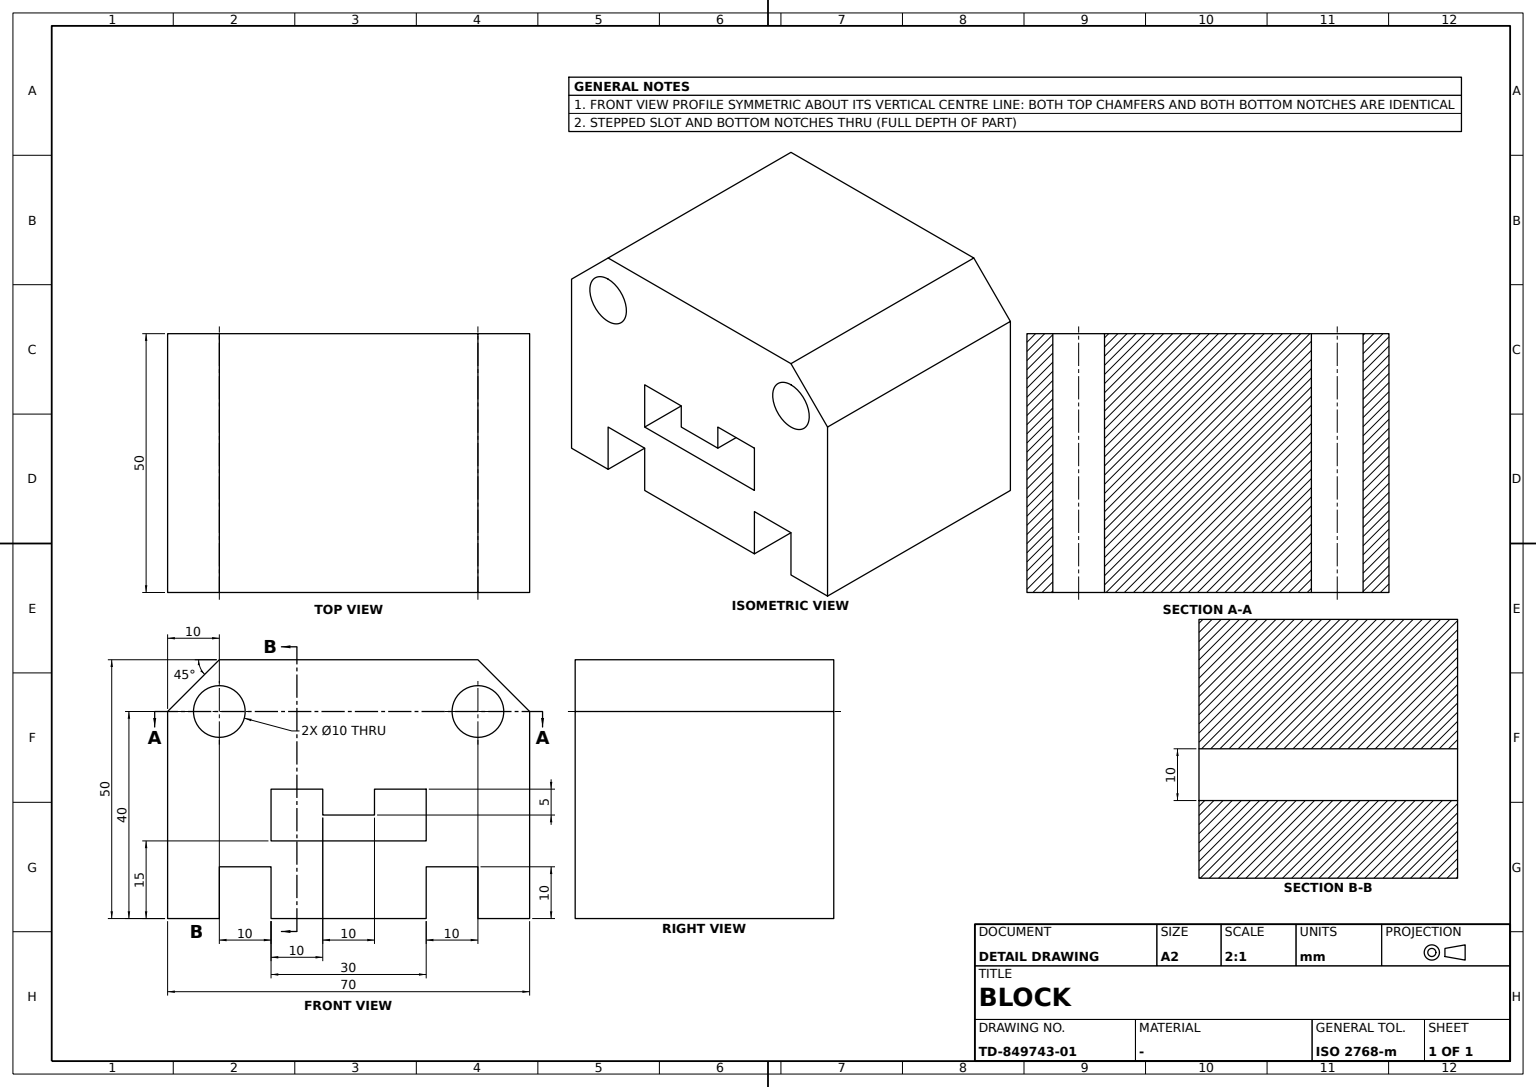
ISO-10303-21;
HEADER;
FILE_DESCRIPTION((''),'2;1');
FILE_NAME('','',(''),(''),'','','');
FILE_SCHEMA(('AUTOMOTIVE_DESIGN'));
ENDSEC;
DATA;
#1=APPLICATION_CONTEXT('');
#2=PRODUCT_CONTEXT('',#1,'mechanical');
#3=PRODUCT('','','',(#2));
#4=PRODUCT_DEFINITION_FORMATION('','',#3);
#5=PRODUCT_DEFINITION_CONTEXT('',#1,'design');
#6=PRODUCT_DEFINITION('','',#4,#5);
#7=PRODUCT_DEFINITION_SHAPE('','',#6);
#8=(LENGTH_UNIT()NAMED_UNIT(*)SI_UNIT(.MILLI.,.METRE.));
#9=(NAMED_UNIT(*)PLANE_ANGLE_UNIT()SI_UNIT($,.RADIAN.));
#10=(NAMED_UNIT(*)SI_UNIT($,.STERADIAN.)SOLID_ANGLE_UNIT());
#11=UNCERTAINTY_MEASURE_WITH_UNIT(LENGTH_MEASURE(0.005),#8,'distance_accuracy_value','');
#12=(GEOMETRIC_REPRESENTATION_CONTEXT(3)GLOBAL_UNCERTAINTY_ASSIGNED_CONTEXT((#11))GLOBAL_UNIT_ASSIGNED_CONTEXT((#8,#9,#10))REPRESENTATION_CONTEXT('',''));
#13=CARTESIAN_POINT('',(-35.,25.,0.));
#14=VERTEX_POINT('',#13);
#15=CARTESIAN_POINT('',(-35.,-25.,0.));
#16=VERTEX_POINT('',#15);
#17=CARTESIAN_POINT('',(-35.,0.,0.));
#18=DIRECTION('',(0.,-1.,0.));
#19=VECTOR('',#18,1000.);
#20=LINE('',#17,#19);
#21=EDGE_CURVE('',#14,#16,#20,.T.);
#22=ORIENTED_EDGE('',*,*,#21,.F.);
#23=CARTESIAN_POINT('',(-25.,25.,0.));
#24=VERTEX_POINT('',#23);
#25=CARTESIAN_POINT('',(0.,25.,0.));
#26=DIRECTION('',(1.,0.,0.));
#27=VECTOR('',#26,1000.);
#28=LINE('',#25,#27);
#29=EDGE_CURVE('',#14,#24,#28,.T.);
#30=ORIENTED_EDGE('',*,*,#29,.T.);
#31=CARTESIAN_POINT('',(-25.,-25.,0.));
#32=VERTEX_POINT('',#31);
#33=CARTESIAN_POINT('',(-25.,0.,0.));
#34=LINE('',#33,#19);
#35=EDGE_CURVE('',#24,#32,#34,.T.);
#36=ORIENTED_EDGE('',*,*,#35,.T.);
#37=CARTESIAN_POINT('',(0.,-25.,0.));
#38=DIRECTION('',(-1.,0.,0.));
#39=VECTOR('',#38,1000.);
#40=LINE('',#37,#39);
#41=EDGE_CURVE('',#32,#16,#40,.T.);
#42=ORIENTED_EDGE('',*,*,#41,.T.);
#43=EDGE_LOOP('',(#22,#30,#36,#42));
#44=FACE_BOUND('',#43,.T.);
#45=CARTESIAN_POINT('',(0.,0.,0.));
#46=DIRECTION('',(0.,0.,1.));
#47=AXIS2_PLACEMENT_3D('',#45,#46,#26);
#48=PLANE('',#47);
#49=ADVANCED_FACE('',(#44),#48,.F.);
#50=CARTESIAN_POINT('',(-15.,25.,15.));
#51=VERTEX_POINT('',#50);
#52=CARTESIAN_POINT('',(-15.,25.,25.));
#53=VERTEX_POINT('',#52);
#54=CARTESIAN_POINT('',(-15.,25.,0.));
#55=VECTOR('',#46,1000.);
#56=LINE('',#54,#55);
#57=EDGE_CURVE('',#51,#53,#56,.T.);
#58=ORIENTED_EDGE('',*,*,#57,.T.);
#59=CARTESIAN_POINT('',(-15.,-25.,25.));
#60=VERTEX_POINT('',#59);
#61=LINE('',#52,#19);
#62=EDGE_CURVE('',#53,#60,#61,.T.);
#63=ORIENTED_EDGE('',*,*,#62,.T.);
#64=CARTESIAN_POINT('',(-15.,-25.,15.));
#65=VERTEX_POINT('',#64);
#66=CARTESIAN_POINT('',(-15.,-25.,0.));
#67=LINE('',#66,#55);
#68=EDGE_CURVE('',#65,#60,#67,.T.);
#69=ORIENTED_EDGE('',*,*,#68,.F.);
#70=LINE('',#50,#19);
#71=EDGE_CURVE('',#51,#65,#70,.T.);
#72=ORIENTED_EDGE('',*,*,#71,.F.);
#73=EDGE_LOOP('',(#58,#63,#69,#72));
#74=FACE_BOUND('',#73,.T.);
#75=AXIS2_PLACEMENT_3D('',#54,#26,#46);
#76=PLANE('',#75);
#77=ADVANCED_FACE('',(#74),#76,.T.);
#78=CARTESIAN_POINT('',(-5.,-25.,25.));
#79=VERTEX_POINT('',#78);
#80=CARTESIAN_POINT('',(-5.,-25.,20.));
#81=VERTEX_POINT('',#80);
#82=DIRECTION('',(0.,0.,-1.));
#83=VECTOR('',#82,1000.);
#84=LINE('',#78,#83);
#85=EDGE_CURVE('',#79,#81,#84,.T.);
#86=ORIENTED_EDGE('',*,*,#85,.F.);
#87=CARTESIAN_POINT('',(-5.,25.,25.));
#88=VERTEX_POINT('',#87);
#89=LINE('',#87,#19);
#90=EDGE_CURVE('',#88,#79,#89,.T.);
#91=ORIENTED_EDGE('',*,*,#90,.F.);
#92=CARTESIAN_POINT('',(-5.,25.,20.));
#93=VERTEX_POINT('',#92);
#94=CARTESIAN_POINT('',(-5.,25.,0.));
#95=LINE('',#94,#83);
#96=EDGE_CURVE('',#88,#93,#95,.T.);
#97=ORIENTED_EDGE('',*,*,#96,.T.);
#98=LINE('',#92,#19);
#99=EDGE_CURVE('',#93,#81,#98,.T.);
#100=ORIENTED_EDGE('',*,*,#99,.T.);
#101=EDGE_LOOP('',(#86,#91,#97,#100));
#102=FACE_BOUND('',#101,.T.);
#103=AXIS2_PLACEMENT_3D('',#87,#38,#82);
#104=PLANE('',#103);
#105=ADVANCED_FACE('',(#102),#104,.T.);
#106=VERTEX_POINT('',#54);
#107=VERTEX_POINT('',#66);
#108=LINE('',#54,#19);
#109=EDGE_CURVE('',#106,#107,#108,.T.);
#110=ORIENTED_EDGE('',*,*,#109,.T.);
#111=CARTESIAN_POINT('',(-15.,-25.,10.));
#112=VERTEX_POINT('',#111);
#113=EDGE_CURVE('',#107,#112,#67,.T.);
#114=ORIENTED_EDGE('',*,*,#113,.T.);
#115=CARTESIAN_POINT('',(-15.,25.,10.));
#116=VERTEX_POINT('',#115);
#117=LINE('',#115,#19);
#118=EDGE_CURVE('',#116,#112,#117,.T.);
#119=ORIENTED_EDGE('',*,*,#118,.F.);
#120=EDGE_CURVE('',#106,#116,#56,.T.);
#121=ORIENTED_EDGE('',*,*,#120,.F.);
#122=EDGE_LOOP('',(#110,#114,#119,#121));
#123=FACE_BOUND('',#122,.T.);
#124=ADVANCED_FACE('',(#123),#76,.F.);
#125=CARTESIAN_POINT('',(25.,25.,50.));
#126=VERTEX_POINT('',#125);
#127=CARTESIAN_POINT('',(35.,25.,40.));
#128=VERTEX_POINT('',#127);
#129=CARTESIAN_POINT('',(20.,25.,55.));
#130=DIRECTION('',(0.707106781,0.,-0.707106781));
#131=VECTOR('',#130,1000.);
#132=LINE('',#129,#131);
#133=EDGE_CURVE('',#126,#128,#132,.T.);
#134=ORIENTED_EDGE('',*,*,#133,.F.);
#135=CARTESIAN_POINT('',(25.,-25.,50.));
#136=VERTEX_POINT('',#135);
#137=CARTESIAN_POINT('',(25.,0.,50.));
#138=LINE('',#137,#19);
#139=EDGE_CURVE('',#126,#136,#138,.T.);
#140=ORIENTED_EDGE('',*,*,#139,.T.);
#141=CARTESIAN_POINT('',(35.,-25.,40.));
#142=VERTEX_POINT('',#141);
#143=CARTESIAN_POINT('',(55.,-25.,20.));
#144=DIRECTION('',(-0.707106781,0.,0.707106781));
#145=VECTOR('',#144,1000.);
#146=LINE('',#143,#145);
#147=EDGE_CURVE('',#142,#136,#146,.T.);
#148=ORIENTED_EDGE('',*,*,#147,.F.);
#149=CARTESIAN_POINT('',(35.,35.,40.));
#150=LINE('',#149,#19);
#151=EDGE_CURVE('',#128,#142,#150,.T.);
#152=ORIENTED_EDGE('',*,*,#151,.F.);
#153=EDGE_LOOP('',(#134,#140,#148,#152));
#154=FACE_BOUND('',#153,.T.);
#155=DIRECTION('',(-0.707106781,0.,-0.707106781));
#156=AXIS2_PLACEMENT_3D('',#149,#155,#18);
#157=PLANE('',#156);
#158=ADVANCED_FACE('',(#154),#157,.F.);
#159=CARTESIAN_POINT('',(25.,25.,0.));
#160=VERTEX_POINT('',#159);
#161=CARTESIAN_POINT('',(35.,25.,0.));
#162=VERTEX_POINT('',#161);
#163=EDGE_CURVE('',#160,#162,#28,.T.);
#164=ORIENTED_EDGE('',*,*,#163,.T.);
#165=CARTESIAN_POINT('',(35.,-25.,0.));
#166=VERTEX_POINT('',#165);
#167=CARTESIAN_POINT('',(35.,0.,0.));
#168=DIRECTION('',(0.,1.,0.));
#169=VECTOR('',#168,1000.);
#170=LINE('',#167,#169);
#171=EDGE_CURVE('',#166,#162,#170,.T.);
#172=ORIENTED_EDGE('',*,*,#171,.F.);
#173=CARTESIAN_POINT('',(25.,-25.,0.));
#174=VERTEX_POINT('',#173);
#175=EDGE_CURVE('',#166,#174,#40,.T.);
#176=ORIENTED_EDGE('',*,*,#175,.T.);
#177=LINE('',#159,#19);
#178=EDGE_CURVE('',#160,#174,#177,.T.);
#179=ORIENTED_EDGE('',*,*,#178,.F.);
#180=EDGE_LOOP('',(#164,#172,#176,#179));
#181=FACE_BOUND('',#180,.T.);
#182=ADVANCED_FACE('',(#181),#48,.F.);
#183=CARTESIAN_POINT('',(-25.,25.,10.));
#184=VERTEX_POINT('',#183);
#185=CARTESIAN_POINT('',(-25.,-25.,10.));
#186=VERTEX_POINT('',#185);
#187=LINE('',#183,#19);
#188=EDGE_CURVE('',#184,#186,#187,.T.);
#189=ORIENTED_EDGE('',*,*,#188,.F.);
#190=CARTESIAN_POINT('',(-35.,25.,10.));
#191=LINE('',#190,#39);
#192=EDGE_CURVE('',#116,#184,#191,.T.);
#193=ORIENTED_EDGE('',*,*,#192,.F.);
#194=ORIENTED_EDGE('',*,*,#118,.T.);
#195=CARTESIAN_POINT('',(25.,-25.,10.));
#196=LINE('',#195,#39);
#197=EDGE_CURVE('',#112,#186,#196,.T.);
#198=ORIENTED_EDGE('',*,*,#197,.T.);
#199=EDGE_LOOP('',(#189,#193,#194,#198));
#200=FACE_BOUND('',#199,.T.);
#201=CARTESIAN_POINT('',(25.,25.,10.));
#202=AXIS2_PLACEMENT_3D('',#201,#46,#38);
#203=PLANE('',#202);
#204=ADVANCED_FACE('',(#200),#203,.F.);
#205=CARTESIAN_POINT('',(-35.,25.,40.));
#206=VERTEX_POINT('',#205);
#207=CARTESIAN_POINT('',(-25.,25.,50.));
#208=VERTEX_POINT('',#207);
#209=CARTESIAN_POINT('',(-55.,25.,20.));
#210=DIRECTION('',(0.707106781,0.,0.707106781));
#211=VECTOR('',#210,1000.);
#212=LINE('',#209,#211);
#213=EDGE_CURVE('',#206,#208,#212,.T.);
#214=ORIENTED_EDGE('',*,*,#213,.F.);
#215=CARTESIAN_POINT('',(-35.,-25.,40.));
#216=VERTEX_POINT('',#215);
#217=CARTESIAN_POINT('',(-35.,-35.,40.));
#218=LINE('',#217,#169);
#219=EDGE_CURVE('',#216,#206,#218,.T.);
#220=ORIENTED_EDGE('',*,*,#219,.F.);
#221=CARTESIAN_POINT('',(-25.,-25.,50.));
#222=VERTEX_POINT('',#221);
#223=CARTESIAN_POINT('',(-20.,-25.,55.));
#224=VECTOR('',#155,1000.);
#225=LINE('',#223,#224);
#226=EDGE_CURVE('',#222,#216,#225,.T.);
#227=ORIENTED_EDGE('',*,*,#226,.F.);
#228=CARTESIAN_POINT('',(-25.,0.,50.));
#229=LINE('',#228,#169);
#230=EDGE_CURVE('',#222,#208,#229,.T.);
#231=ORIENTED_EDGE('',*,*,#230,.T.);
#232=EDGE_LOOP('',(#214,#220,#227,#231));
#233=FACE_BOUND('',#232,.T.);
#234=AXIS2_PLACEMENT_3D('',#217,#130,#168);
#235=PLANE('',#234);
#236=ADVANCED_FACE('',(#233),#235,.F.);
#237=CARTESIAN_POINT('',(5.,25.,25.));
#238=VERTEX_POINT('',#237);
#239=CARTESIAN_POINT('',(5.,-25.,25.));
#240=VERTEX_POINT('',#239);
#241=LINE('',#237,#19);
#242=EDGE_CURVE('',#238,#240,#241,.T.);
#243=ORIENTED_EDGE('',*,*,#242,.F.);
#244=CARTESIAN_POINT('',(15.,25.,25.));
#245=VERTEX_POINT('',#244);
#246=CARTESIAN_POINT('',(-35.,25.,25.));
#247=LINE('',#246,#27);
#248=EDGE_CURVE('',#238,#245,#247,.T.);
#249=ORIENTED_EDGE('',*,*,#248,.T.);
#250=CARTESIAN_POINT('',(15.,-25.,25.));
#251=VERTEX_POINT('',#250);
#252=LINE('',#244,#19);
#253=EDGE_CURVE('',#245,#251,#252,.T.);
#254=ORIENTED_EDGE('',*,*,#253,.T.);
#255=LINE('',#59,#27);
#256=EDGE_CURVE('',#240,#251,#255,.T.);
#257=ORIENTED_EDGE('',*,*,#256,.F.);
#258=EDGE_LOOP('',(#243,#249,#254,#257));
#259=FACE_BOUND('',#258,.T.);
#260=AXIS2_PLACEMENT_3D('',#52,#82,#26);
#261=PLANE('',#260);
#262=ADVANCED_FACE('',(#259),#261,.T.);
#263=EDGE_CURVE('',#53,#88,#247,.T.);
#264=ORIENTED_EDGE('',*,*,#263,.F.);
#265=ORIENTED_EDGE('',*,*,#57,.F.);
#266=CARTESIAN_POINT('',(15.,25.,15.));
#267=VERTEX_POINT('',#266);
#268=CARTESIAN_POINT('',(-35.,25.,15.));
#269=LINE('',#268,#39);
#270=EDGE_CURVE('',#267,#51,#269,.T.);
#271=ORIENTED_EDGE('',*,*,#270,.F.);
#272=CARTESIAN_POINT('',(15.,25.,0.));
#273=LINE('',#272,#83);
#274=EDGE_CURVE('',#245,#267,#273,.T.);
#275=ORIENTED_EDGE('',*,*,#274,.F.);
#276=ORIENTED_EDGE('',*,*,#248,.F.);
#277=CARTESIAN_POINT('',(5.,25.,20.));
#278=VERTEX_POINT('',#277);
#279=CARTESIAN_POINT('',(5.,25.,0.));
#280=LINE('',#279,#55);
#281=EDGE_CURVE('',#278,#238,#280,.T.);
#282=ORIENTED_EDGE('',*,*,#281,.F.);
#283=CARTESIAN_POINT('',(-35.,25.,20.));
#284=LINE('',#283,#27);
#285=EDGE_CURVE('',#93,#278,#284,.T.);
#286=ORIENTED_EDGE('',*,*,#285,.F.);
#287=ORIENTED_EDGE('',*,*,#96,.F.);
#288=EDGE_LOOP('',(#264,#265,#271,#275,#276,#282,#286,#287));
#289=FACE_BOUND('',#288,.T.);
#290=CARTESIAN_POINT('',(-25.,25.,35.));
#291=VERTEX_POINT('',#290);
#292=CARTESIAN_POINT('',(-25.,25.,40.));
#293=AXIS2_PLACEMENT_3D('',#292,#18,#82);
#294=CIRCLE('',#293,5.);
#295=EDGE_CURVE('',#291,#291,#294,.F.);
#296=ORIENTED_EDGE('',*,*,#295,.F.);
#297=EDGE_LOOP('',(#296));
#298=FACE_BOUND('',#297,.T.);
#299=VERTEX_POINT('',#272);
#300=EDGE_CURVE('',#106,#299,#28,.T.);
#301=ORIENTED_EDGE('',*,*,#300,.F.);
#302=ORIENTED_EDGE('',*,*,#120,.T.);
#303=ORIENTED_EDGE('',*,*,#192,.T.);
#304=LINE('',#23,#83);
#305=EDGE_CURVE('',#184,#24,#304,.T.);
#306=ORIENTED_EDGE('',*,*,#305,.T.);
#307=ORIENTED_EDGE('',*,*,#29,.F.);
#308=LINE('',#13,#55);
#309=EDGE_CURVE('',#14,#206,#308,.T.);
#310=ORIENTED_EDGE('',*,*,#309,.T.);
#311=ORIENTED_EDGE('',*,*,#213,.T.);
#312=CARTESIAN_POINT('',(0.,25.,50.));
#313=LINE('',#312,#27);
#314=EDGE_CURVE('',#208,#126,#313,.T.);
#315=ORIENTED_EDGE('',*,*,#314,.T.);
#316=ORIENTED_EDGE('',*,*,#133,.T.);
#317=LINE('',#161,#55);
#318=EDGE_CURVE('',#162,#128,#317,.T.);
#319=ORIENTED_EDGE('',*,*,#318,.F.);
#320=ORIENTED_EDGE('',*,*,#163,.F.);
#321=VERTEX_POINT('',#201);
#322=LINE('',#159,#55);
#323=EDGE_CURVE('',#160,#321,#322,.T.);
#324=ORIENTED_EDGE('',*,*,#323,.T.);
#325=CARTESIAN_POINT('',(15.,25.,10.));
#326=VERTEX_POINT('',#325);
#327=EDGE_CURVE('',#321,#326,#191,.T.);
#328=ORIENTED_EDGE('',*,*,#327,.T.);
#329=EDGE_CURVE('',#326,#299,#273,.T.);
#330=ORIENTED_EDGE('',*,*,#329,.T.);
#331=EDGE_LOOP('',(#301,#302,#303,#306,#307,#310,#311,#315,#316,#319,#320,#324,#328,#330));
#332=FACE_BOUND('',#331,.T.);
#333=CARTESIAN_POINT('',(25.,25.,35.));
#334=VERTEX_POINT('',#333);
#335=CARTESIAN_POINT('',(25.,25.,40.));
#336=AXIS2_PLACEMENT_3D('',#335,#18,#82);
#337=CIRCLE('',#336,5.);
#338=EDGE_CURVE('',#334,#334,#337,.F.);
#339=ORIENTED_EDGE('',*,*,#338,.F.);
#340=EDGE_LOOP('',(#339));
#341=FACE_BOUND('',#340,.T.);
#342=AXIS2_PLACEMENT_3D('',#13,#18,#26);
#343=PLANE('',#342);
#344=ADVANCED_FACE('',(#289,#298,#332,#341),#343,.F.);
#345=VERTEX_POINT('',#195);
#346=CARTESIAN_POINT('',(15.,-25.,10.));
#347=VERTEX_POINT('',#346);
#348=EDGE_CURVE('',#345,#347,#196,.T.);
#349=ORIENTED_EDGE('',*,*,#348,.T.);
#350=LINE('',#325,#19);
#351=EDGE_CURVE('',#326,#347,#350,.T.);
#352=ORIENTED_EDGE('',*,*,#351,.F.);
#353=ORIENTED_EDGE('',*,*,#327,.F.);
#354=LINE('',#201,#19);
#355=EDGE_CURVE('',#321,#345,#354,.T.);
#356=ORIENTED_EDGE('',*,*,#355,.T.);
#357=EDGE_LOOP('',(#349,#352,#353,#356));
#358=FACE_BOUND('',#357,.T.);
#359=ADVANCED_FACE('',(#358),#203,.F.);
#360=CARTESIAN_POINT('',(-25.,-25.,45.));
#361=VERTEX_POINT('',#360);
#362=CARTESIAN_POINT('',(-25.,-25.,40.));
#363=AXIS2_PLACEMENT_3D('',#362,#168,#46);
#364=CIRCLE('',#363,5.);
#365=EDGE_CURVE('',#361,#361,#364,.T.);
#366=ORIENTED_EDGE('',*,*,#365,.F.);
#367=EDGE_LOOP('',(#366));
#368=FACE_BOUND('',#367,.T.);
#369=ORIENTED_EDGE('',*,*,#295,.T.);
#370=EDGE_LOOP('',(#369));
#371=FACE_BOUND('',#370,.T.);
#372=CARTESIAN_POINT('',(-25.,-0.66,40.));
#373=AXIS2_PLACEMENT_3D('',#372,#168,#38);
#374=CYLINDRICAL_SURFACE('',#373,5.);
#375=ADVANCED_FACE('',(#368,#371),#374,.F.);
#376=ORIENTED_EDGE('',*,*,#263,.T.);
#377=ORIENTED_EDGE('',*,*,#90,.T.);
#378=EDGE_CURVE('',#60,#79,#255,.T.);
#379=ORIENTED_EDGE('',*,*,#378,.F.);
#380=ORIENTED_EDGE('',*,*,#62,.F.);
#381=EDGE_LOOP('',(#376,#377,#379,#380));
#382=FACE_BOUND('',#381,.T.);
#383=ADVANCED_FACE('',(#382),#261,.T.);
#384=CARTESIAN_POINT('',(15.,-25.,0.));
#385=VERTEX_POINT('',#384);
#386=LINE('',#384,#55);
#387=EDGE_CURVE('',#385,#347,#386,.T.);
#388=ORIENTED_EDGE('',*,*,#387,.F.);
#389=CARTESIAN_POINT('',(15.,0.,0.));
#390=LINE('',#389,#19);
#391=EDGE_CURVE('',#299,#385,#390,.T.);
#392=ORIENTED_EDGE('',*,*,#391,.F.);
#393=ORIENTED_EDGE('',*,*,#329,.F.);
#394=ORIENTED_EDGE('',*,*,#351,.T.);
#395=EDGE_LOOP('',(#388,#392,#393,#394));
#396=FACE_BOUND('',#395,.T.);
#397=AXIS2_PLACEMENT_3D('',#325,#38,#82);
#398=PLANE('',#397);
#399=ADVANCED_FACE('',(#396),#398,.F.);
#400=ORIENTED_EDGE('',*,*,#171,.T.);
#401=ORIENTED_EDGE('',*,*,#318,.T.);
#402=ORIENTED_EDGE('',*,*,#151,.T.);
#403=LINE('',#165,#55);
#404=EDGE_CURVE('',#166,#142,#403,.T.);
#405=ORIENTED_EDGE('',*,*,#404,.F.);
#406=EDGE_LOOP('',(#400,#401,#402,#405));
#407=FACE_BOUND('',#406,.T.);
#408=AXIS2_PLACEMENT_3D('',#165,#26,#168);
#409=PLANE('',#408);
#410=ADVANCED_FACE('',(#407),#409,.T.);
#411=ORIENTED_EDGE('',*,*,#305,.F.);
#412=ORIENTED_EDGE('',*,*,#188,.T.);
#413=LINE('',#31,#55);
#414=EDGE_CURVE('',#32,#186,#413,.T.);
#415=ORIENTED_EDGE('',*,*,#414,.F.);
#416=ORIENTED_EDGE('',*,*,#35,.F.);
#417=EDGE_LOOP('',(#411,#412,#415,#416));
#418=FACE_BOUND('',#417,.T.);
#419=AXIS2_PLACEMENT_3D('',#183,#38,#82);
#420=PLANE('',#419);
#421=ADVANCED_FACE('',(#418),#420,.F.);
#422=ORIENTED_EDGE('',*,*,#274,.T.);
#423=CARTESIAN_POINT('',(15.,-25.,15.));
#424=VERTEX_POINT('',#423);
#425=LINE('',#266,#19);
#426=EDGE_CURVE('',#267,#424,#425,.T.);
#427=ORIENTED_EDGE('',*,*,#426,.T.);
#428=LINE('',#346,#83);
#429=EDGE_CURVE('',#251,#424,#428,.T.);
#430=ORIENTED_EDGE('',*,*,#429,.F.);
#431=ORIENTED_EDGE('',*,*,#253,.F.);
#432=EDGE_LOOP('',(#422,#427,#430,#431));
#433=FACE_BOUND('',#432,.T.);
#434=ADVANCED_FACE('',(#433),#398,.T.);
#435=ORIENTED_EDGE('',*,*,#219,.T.);
#436=ORIENTED_EDGE('',*,*,#309,.F.);
#437=ORIENTED_EDGE('',*,*,#21,.T.);
#438=LINE('',#15,#55);
#439=EDGE_CURVE('',#16,#216,#438,.T.);
#440=ORIENTED_EDGE('',*,*,#439,.T.);
#441=EDGE_LOOP('',(#435,#436,#437,#440));
#442=FACE_BOUND('',#441,.T.);
#443=AXIS2_PLACEMENT_3D('',#13,#38,#18);
#444=PLANE('',#443);
#445=ADVANCED_FACE('',(#442),#444,.T.);
#446=ORIENTED_EDGE('',*,*,#270,.T.);
#447=ORIENTED_EDGE('',*,*,#71,.T.);
#448=LINE('',#423,#39);
#449=EDGE_CURVE('',#424,#65,#448,.T.);
#450=ORIENTED_EDGE('',*,*,#449,.F.);
#451=ORIENTED_EDGE('',*,*,#426,.F.);
#452=EDGE_LOOP('',(#446,#447,#450,#451));
#453=FACE_BOUND('',#452,.T.);
#454=AXIS2_PLACEMENT_3D('',#266,#46,#38);
#455=PLANE('',#454);
#456=ADVANCED_FACE('',(#453),#455,.T.);
#457=ORIENTED_EDGE('',*,*,#139,.F.);
#458=ORIENTED_EDGE('',*,*,#314,.F.);
#459=ORIENTED_EDGE('',*,*,#230,.F.);
#460=CARTESIAN_POINT('',(0.,-25.,50.));
#461=LINE('',#460,#39);
#462=EDGE_CURVE('',#136,#222,#461,.T.);
#463=ORIENTED_EDGE('',*,*,#462,.F.);
#464=EDGE_LOOP('',(#457,#458,#459,#463));
#465=FACE_BOUND('',#464,.T.);
#466=CARTESIAN_POINT('',(0.,0.,50.));
#467=AXIS2_PLACEMENT_3D('',#466,#46,#26);
#468=PLANE('',#467);
#469=ADVANCED_FACE('',(#465),#468,.T.);
#470=CARTESIAN_POINT('',(25.,-25.,45.));
#471=VERTEX_POINT('',#470);
#472=CARTESIAN_POINT('',(25.,-25.,40.));
#473=AXIS2_PLACEMENT_3D('',#472,#168,#46);
#474=CIRCLE('',#473,5.);
#475=EDGE_CURVE('',#471,#471,#474,.T.);
#476=ORIENTED_EDGE('',*,*,#475,.T.);
#477=EDGE_LOOP('',(#476));
#478=FACE_BOUND('',#477,.T.);
#479=ORIENTED_EDGE('',*,*,#348,.F.);
#480=LINE('',#173,#55);
#481=EDGE_CURVE('',#174,#345,#480,.T.);
#482=ORIENTED_EDGE('',*,*,#481,.F.);
#483=ORIENTED_EDGE('',*,*,#175,.F.);
#484=ORIENTED_EDGE('',*,*,#404,.T.);
#485=ORIENTED_EDGE('',*,*,#147,.T.);
#486=ORIENTED_EDGE('',*,*,#462,.T.);
#487=ORIENTED_EDGE('',*,*,#226,.T.);
#488=ORIENTED_EDGE('',*,*,#439,.F.);
#489=ORIENTED_EDGE('',*,*,#41,.F.);
#490=ORIENTED_EDGE('',*,*,#414,.T.);
#491=ORIENTED_EDGE('',*,*,#197,.F.);
#492=ORIENTED_EDGE('',*,*,#113,.F.);
#493=EDGE_CURVE('',#385,#107,#40,.T.);
#494=ORIENTED_EDGE('',*,*,#493,.F.);
#495=ORIENTED_EDGE('',*,*,#387,.T.);
#496=EDGE_LOOP('',(#479,#482,#483,#484,#485,#486,#487,#488,#489,#490,#491,#492,#494,#495));
#497=FACE_BOUND('',#496,.T.);
#498=CARTESIAN_POINT('',(5.,-25.,20.));
#499=VERTEX_POINT('',#498);
#500=LINE('',#498,#55);
#501=EDGE_CURVE('',#499,#240,#500,.T.);
#502=ORIENTED_EDGE('',*,*,#501,.T.);
#503=ORIENTED_EDGE('',*,*,#256,.T.);
#504=ORIENTED_EDGE('',*,*,#429,.T.);
#505=ORIENTED_EDGE('',*,*,#449,.T.);
#506=ORIENTED_EDGE('',*,*,#68,.T.);
#507=ORIENTED_EDGE('',*,*,#378,.T.);
#508=ORIENTED_EDGE('',*,*,#85,.T.);
#509=LINE('',#80,#27);
#510=EDGE_CURVE('',#81,#499,#509,.T.);
#511=ORIENTED_EDGE('',*,*,#510,.T.);
#512=EDGE_LOOP('',(#502,#503,#504,#505,#506,#507,#508,#511));
#513=FACE_BOUND('',#512,.T.);
#514=ORIENTED_EDGE('',*,*,#365,.T.);
#515=EDGE_LOOP('',(#514));
#516=FACE_BOUND('',#515,.T.);
#517=AXIS2_PLACEMENT_3D('',#165,#168,#38);
#518=PLANE('',#517);
#519=ADVANCED_FACE('',(#478,#497,#513,#516),#518,.F.);
#520=ORIENTED_EDGE('',*,*,#501,.F.);
#521=LINE('',#277,#19);
#522=EDGE_CURVE('',#278,#499,#521,.T.);
#523=ORIENTED_EDGE('',*,*,#522,.F.);
#524=ORIENTED_EDGE('',*,*,#281,.T.);
#525=ORIENTED_EDGE('',*,*,#242,.T.);
#526=EDGE_LOOP('',(#520,#523,#524,#525));
#527=FACE_BOUND('',#526,.T.);
#528=AXIS2_PLACEMENT_3D('',#277,#26,#46);
#529=PLANE('',#528);
#530=ADVANCED_FACE('',(#527),#529,.T.);
#531=ORIENTED_EDGE('',*,*,#338,.T.);
#532=EDGE_LOOP('',(#531));
#533=FACE_BOUND('',#532,.T.);
#534=ORIENTED_EDGE('',*,*,#475,.F.);
#535=EDGE_LOOP('',(#534));
#536=FACE_BOUND('',#535,.T.);
#537=CARTESIAN_POINT('',(25.,-0.66,40.));
#538=AXIS2_PLACEMENT_3D('',#537,#168,#38);
#539=CYLINDRICAL_SURFACE('',#538,5.);
#540=ADVANCED_FACE('',(#533,#536),#539,.F.);
#541=ORIENTED_EDGE('',*,*,#355,.F.);
#542=ORIENTED_EDGE('',*,*,#323,.F.);
#543=ORIENTED_EDGE('',*,*,#178,.T.);
#544=ORIENTED_EDGE('',*,*,#481,.T.);
#545=EDGE_LOOP('',(#541,#542,#543,#544));
#546=FACE_BOUND('',#545,.T.);
#547=AXIS2_PLACEMENT_3D('',#159,#26,#46);
#548=PLANE('',#547);
#549=ADVANCED_FACE('',(#546),#548,.F.);
#550=ORIENTED_EDGE('',*,*,#99,.F.);
#551=ORIENTED_EDGE('',*,*,#285,.T.);
#552=ORIENTED_EDGE('',*,*,#522,.T.);
#553=ORIENTED_EDGE('',*,*,#510,.F.);
#554=EDGE_LOOP('',(#550,#551,#552,#553));
#555=FACE_BOUND('',#554,.T.);
#556=AXIS2_PLACEMENT_3D('',#92,#82,#26);
#557=PLANE('',#556);
#558=ADVANCED_FACE('',(#555),#557,.T.);
#559=ORIENTED_EDGE('',*,*,#493,.T.);
#560=ORIENTED_EDGE('',*,*,#109,.F.);
#561=ORIENTED_EDGE('',*,*,#300,.T.);
#562=ORIENTED_EDGE('',*,*,#391,.T.);
#563=EDGE_LOOP('',(#559,#560,#561,#562));
#564=FACE_BOUND('',#563,.T.);
#565=ADVANCED_FACE('',(#564),#48,.F.);
#566=CLOSED_SHELL('',(#49,#77,#105,#124,#158,#182,#204,#236,#262,#344,#359,#375,#383,#399,#410,#421,#434,#445,#456,#469,#519,#530,#540,#549,#558,#565));
#567=MANIFOLD_SOLID_BREP('',#566);
#568=ADVANCED_BREP_SHAPE_REPRESENTATION('',(#567),#12);
#569=SHAPE_DEFINITION_REPRESENTATION(#7,#568);
ENDSEC;
END-ISO-10303-21;
